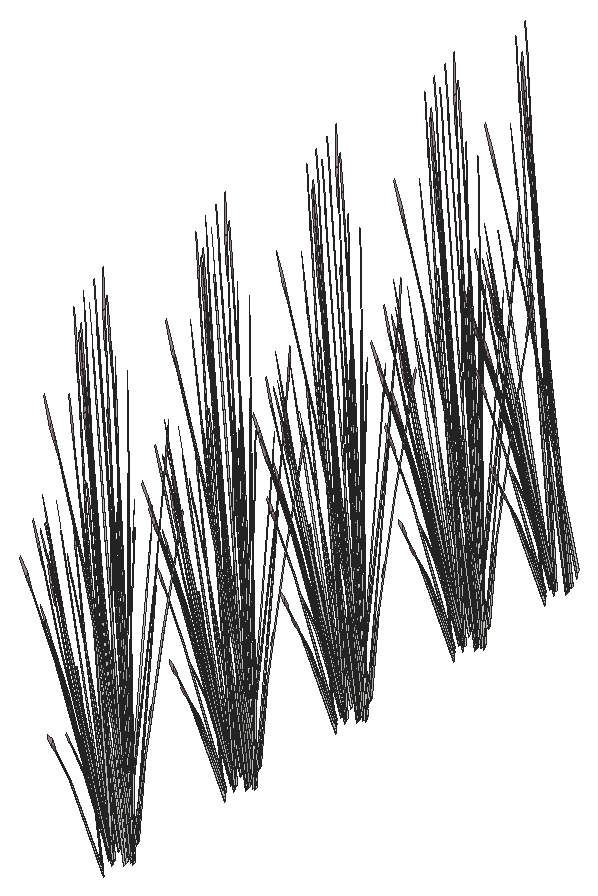
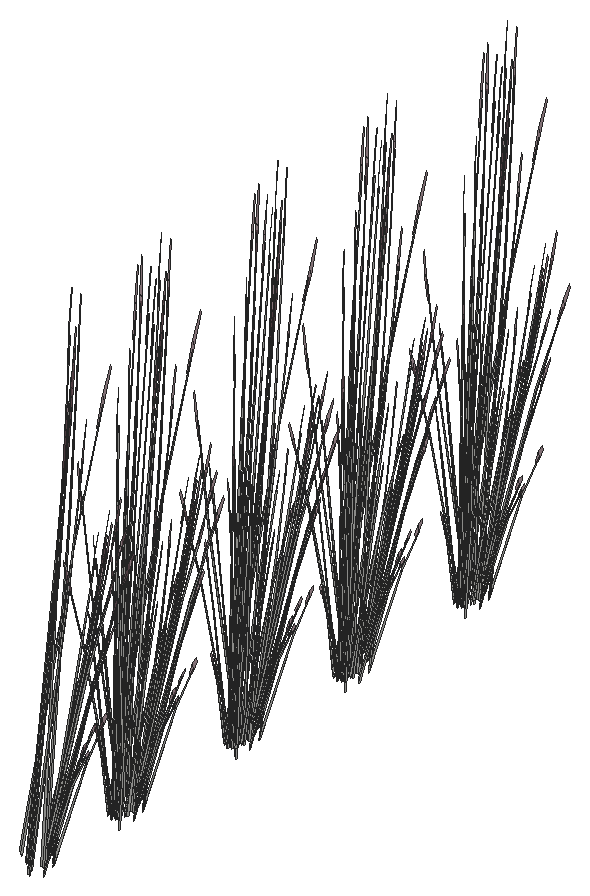
# SketchUp Ruby script. Lengths in inches.
U = 1.inch
M = Sketchup.active_model
def pt(a) = Geom::Point3d.new(a.map { |v| v * U })
def face(e, loops, mat)
  f = e.add_face(loops[0].map { |a| pt(a) })
  loops[1..].each { |l| e.add_face(l.map { |a| pt(a) }).erase! }
  f.material = f.back_material = mat if mat
  f
end
# faces: each face lists its corners as indices into pts; further lists are holes
def faces(e, pts, list, mat = nil) = list.each { |f| face(e, (f[0].is_a?(Array) ? f : [f]).map { |l| l.map { |i| pts[i] } }, mat) }
# xy, xz, yz: faces in a plane at the given z, y or x. An outline is a flat list of corners, or four numbers for a rectangle; further outlines are holes
def ring(l) = l.size == 4 ? [[l[0], l[1]], [l[2], l[1]], [l[2], l[3]], [l[0], l[3]]] : l.each_slice(2).to_a
def flat(e, list, mat, &to3) = list.each { |f| face(e, (f[0].is_a?(Array) ? f : [f]).map { |l| ring(l).map { |u, v| to3.(u, v) } }, mat) }
def xy(e, z, list, mat = nil) = flat(e, list, mat) { |x, y| [x, y, z] }
def xz(e, y, list, mat = nil) = flat(e, list, mat) { |x, z| [x, y, z] }
def yz(e, x, list, mat = nil) = flat(e, list, mat) { |y, z| [x, y, z] }
def lines(e, pts, list) = list.each { |a, b| e.add_line(pt(pts[a]), pt(pts[b])) }
# prism: a flat outline (further loops are holes) pulled along v
def prism(e, loops, v, mat = nil)
  f = face(e, loops, mat); d = Geom::Vector3d.new(v.map { |x| x * U })
  f.pushpull(f.normal.samedirection?(d) ? d.length : -d.length)
end
def box(e, o, s, mat = nil) = prism(e, [[o, [o[0] + s[0], o[1], o[2]], [o[0] + s[0], o[1] + s[1], o[2]], [o[0], o[1] + s[1], o[2]]]], [0, 0, s[2]], mat)
def at(x, y, z, deg = 0) = Geom::Transformation.translation(pt([x, y, z])) * Geom::Transformation.rotation(ORIGIN, Z_AXIS, deg.degrees)
def axes(o, x, y, z) = Geom::Transformation.new([*x, 0, *y, 0, *z, 0, *pt(o).to_a, 1])
def part(name) = M.definitions.add(name)
# library, detail: a bought-in or finely detailed component or shape, given as its bounding box
def library(name, o, s) = part(name).tap { |d| box(d.entities, o, s) }
def detail(e, o, s) = box(e.add_group.entities, o, s)
def put(e, d, t, mat = nil) = e.add_instance(d, t).tap { |i| i.material = mat if mat }
def group(e, t, mat = nil) = e.add_group.tap { |g| g.transformation = t; g.material = mat if mat }.entities
root = M.entities
M.materials.add("LightPink_Translucent").color = [144, 107, 117]
M.materials["LightPink_Translucent"].alpha = 0.75
c1 = part("blade")
p = [[2.15,0.21,22],[0,0.17,0],[0.09,0.45,0],[2.18,0.31,22],[2.29,0.31,22],[0.38,0.45,0],
  [2.48,0.24,33],[2.49,0.24,33],[2.48,0.22,33]]
faces(c1.entities,p,[[0,1,2,3],[4,5,2,3],[6,3,4,7],[8,0,3,6]])
c2 = part("seeds")
p = [[0.3,-0.1,1.38],[-0.01,-0.03,1.59],[-0.01,-0.03,0.03],[0.14,-0.07,-0.07],[0.29,-0.03,3],[0.15,0.01,3.11]]
faces(c2.entities,p,[[0,1,2,3],[1,0,4,5]],"LightPink_Translucent")
c3 = part("blade with seeds")
put(c3.entities,c1,at(0,0,0))
put(c3.entities,c2,axes([2.4,0.25,30.99],[1.5799,-0.05474,1.17369],[-0.12525,1.92788,0.29478],[-0.07173,-0.02425,1.56792]))
put(root,c3,axes([401.51,688.86,4.98],[-0.30095,-0.22541,-0.71045],[0.21388,-0.395,0.08574],[-0.10904,-0.13459,1.00501]))
put(root,c3,axes([401.4,688.56,4.53],[-0.05451,-0.37564,-0.35414],[0.31161,-0.09919,0.4572],[-0.0837,-0.10765,0.87481]))
put(root,c3,axes([400.92,688.49,1.49],[-0.03419,0.06144,1.76342],[-0.3455,0.13246,-0.26939],[-0.08346,-0.12049,0.30037]))
put(root,c3,axes([400.73,689.1,3.875],[0.1311,0.08035,1.71376],[-0.27131,0.33708,0.13857],[-0.16909,-0.15206,0.73262]))
put(root,c3,axes([401.37,688.87,4.68],[-0.34827,0.11086,-0.51099],[-0.06092,-0.41983,-0.3958],[-0.09354,-0.12031,0.97773]))
put(root,c3,axes([402.23,691.41,3.33],[0.305,0.18805,1.51261],[-0.29879,0.40513,0.59816],[-0.13384,-0.24012,1.26806]))
put(root,c3,axes([400.68,689.22,4.53],[-0.20082,-0.29199,-0.35414],[0.2293,-0.2764,0.4572],[-0.1165,-0.04206,0.87481]))
put(root,c3,axes([400.7,688.72,2.13],[-0.10181,0.3808,-0.03893],[-0.31336,-0.11714,-0.17649],[-0.04758,-0.06228,0.58215]))
put(root,c3,axes([400.53,690.46,2.375],[-0.44133,0,0],[0,-0.52122,-0.51607],[0,-0.11871,1.63711]))
put(root,c3,axes([400.61,689.53,2.59],[0.06891,0.12984,1.43002],[-0.15879,0.35293,-0.30754],[-0.16304,-0.08436,0.61141]))
put(root,c3,axes([400.89,689.41,4.98],[-0.35281,-0.01123,-0.71045],[0.0237,-0.47284,0.08574],[-0.14947,-0.0499,1.00501]))
put(root,c3,axes([400.875,690.32,2.33],[-0.32829,0.39208,0.30756],[-0.32849,-0.38796,-0.36492],[-0.01146,-0.11134,1.64885]))
put(root,c3,axes([401.77,691.14,2.4375],[0.09355,-0.55261,-0.23429],[0.44354,0.09633,0.51271],[-0.0775,-0.07631,1.5644]))
put(root,c3,axes([400.78,689.51,4.68],[-0.25628,0.30892,-0.51099],[-0.22444,-0.32634,-0.3958],[-0.13021,-0.047,0.97773]))
put(root,c3,axes([400.2,689.92,2.77],[0.22533,-0.03337,1.1486],[-0.14293,0.29403,0.84392],[-0.11135,-0.04411,0.25299]))
put(root,c3,axes([400.46,689.84,3.875],[0.14639,-0.01056,1.71376],[-0.09712,0.45778,0.13857],[-0.20862,-0.02831,0.73262]))
put(root,c3,axes([401.73,690.92,2.21],[-0.21202,-0.39143,-0.44739],[0.32115,-0.27564,0.21531],[-0.06861,-0.04843,1.43643]))
put(root,c3,axes([401.54,691.07,2.06],[-0.36714,-0.07646,-0.62353],[0.07747,-0.47163,-0.16365],[-0.10956,-0.05715,1.37633]))
put(root,c3,axes([400.36,690.4,1.49],[0.00895,0.0735,1.76342],[-0.18044,0.38382,-0.26939],[-0.12817,-0.01935,0.30037]))
put(root,c3,axes([401.15,691.78,2.03],[-0.08291,-0.40636,-0.30978],[0.32928,-0.11539,0.30978],[-0.06638,-0.04686,1.38974]))
put(root,c3,axes([401.0625,691.96,2.02],[-0.33032,-0.23318,-0.49651],[0.19744,-0.41812,0],[-0.07523,-0.05311,1.57504]))
put(root,c3,axes([400.33,690.23,4.53],[-0.29332,-0.1301,-0.35414],[0.08555,-0.37955,0.4572],[-0.11809,0.0348,0.87481]))
put(root,c3,axes([401.96,691.14,2.67],[-0.35635,0.30962,-0.29095],[-0.23697,-0.43749,-0.50002],[-0.08792,-0.04443,1.59708]))
put(root,c3,axes([401.93,691.27,2.62],[-0.06809,0.4162,0.1448],[-0.33266,-0.07225,-0.41347],[-0.06054,-0.04274,1.26744]))
put(root,c3,axes([401.22,690.17,3.34],[0.10032,-0.06746,1.77064],[0.0346,0.47103,0.13857],[-0.2173,0.0625,0.63284]))
put(root,c3,axes([402.36,691.28,2.46],[-0.34464,-0.37536,-0.25192],[0.29,-0.42149,0.5513],[-0.0928,0.04391,1.68216]))
put(root,c3,axes([401.45,692,2.48],[0.33032,0.23318,0.49651],[-0.19744,0.41812,0],[-0.07523,-0.05311,1.57504]))
put(root,c3,axes([400.53,690.43,4.68],[-0.09562,0.42421,-0.51099],[-0.32782,-0.1454,-0.3958],[-0.13199,0.0389,0.97773]))
put(root,c3,axes([401.26,692.24,2.375],[-0.22066,0.46731,0],[-0.36918,-0.26061,-0.51607],[-0.08408,-0.05936,1.63711]))
put(root,c3,axes([402.1875,691.2,2.21],[-0.38326,0.02879,-0.44739],[-0.03466,-0.47788,0.21531],[-0.06861,0.04843,1.43643]))
put(root,c3,axes([400.52,690.65,3.875],[0.12246,-0.09864,1.71376],[0.1031,0.45582,0.13857],[-0.19225,0.10302,0.73262]))
put(root,c3,axes([400.14,691.42,2.59],[0.12266,0.03828,1.43002],[0.07906,0.39104,-0.30754],[-0.16661,0.0732,0.61141]))
put(root,c3,axes([399.88,692.24,2.77],[0.14709,-0.21136,1.1486],[0.05804,0.3346,0.84392],[-0.1063,0.05991,0.25299]))
put(root,c3,axes([400.43,691.33,4.53],[-0.30722,0.06665,-0.35414],[-0.08112,-0.381,0.4572],[-0.08804,0.10234,0.87481]))
put(root,c3,axes([402.2,691.47,2.06],[-0.23773,0.35053,-0.62353],[-0.29532,-0.31785,-0.16365],[-0.09526,0.08744,1.37633]))
put(root,c3,axes([400.97,690.95,3.875],[0.08815,-0.14329,1.71376],[0.22258,0.38678,0.13857],[-0.15267,0.17614,0.73262]))
put(root,c3,axes([400.6875,691.37,4.68],[0.09067,0.42583,-0.51099],[-0.34336,0.07449,-0.3958],[-0.0984,0.11438,0.97773]))
put(root,c3,axes([400.27,692.46,1.49],[0.04734,0.04659,1.76342],[0.08027,0.4317,-0.26939],[-0.10492,0.09206,0.30037]))
put(root,c3,axes([400.9,691.31,3.875],[0.06572,-0.16029,1.71376],[0.27569,0.33172,0.13857],[-0.12437,0.20675,0.73262]))
put(root,c3,axes([400.98,692.21,4.53],[-0.23881,0.24554,-0.35414],[-0.22606,-0.28036,0.4572],[-0.0344,0.14245,0.87481]))
put(root,c3,axes([401.13,693.16,2.77],[-0.00913,-0.2773,1.1486],[0.22824,0.19778,0.84392],[-0.04489,0.13217,0.25299]))
put(root,c3,axes([401.13,691.95,5.34],[-0.00918,0.43138,-0.7886],[-0.38672,-0.02897,0.09517],[-0.04081,0.18275,1.11556]))
put(root,c3,axes([400.86,692.92,2.59],[0.11138,-0.07357,1.43002],[0.27499,0.22183,-0.30754],[-0.08185,0.19194,0.61141]))
put(root,c3,axes([401.01,692.56,3.36],[0.00775,-0.24075,1.54345],[0.34877,0.12716,0.21329],[-0.03022,0.25658,0.72882]))
put(root,c3,axes([401.27,706.37,3.875],[0.08068,0.14973,1.71376],[-0.3728,0.12606,0.13857],[-0.08426,-0.23506,0.73262]))
put(root,c3,axes([401.17,705.97,2.59],[-0.02137,0.15256,1.43002],[-0.31245,0.12771,-0.30754],[-0.07303,-0.19719,0.61141]))
put(root,c3,axes([401.0625,705.72,2.77],[0.18411,0.16231,1.1486],[-0.26813,0.09757,0.84392],[-0.05737,-0.12474,0.25299]))
put(root,c3,axes([401.51,706.58,4.98],[-0.30095,-0.22541,-0.71045],[0.21388,-0.395,0.08574],[-0.10904,-0.13459,1.00501]))
put(root,c3,axes([401.4,706.29,4.53],[-0.05451,-0.37564,-0.35414],[0.31161,-0.09919,0.4572],[-0.0837,-0.10765,0.87481]))
put(root,c3,axes([400.92,706.21,1.49],[-0.03419,0.06144,1.76342],[-0.3455,0.13246,-0.26939],[-0.08346,-0.12049,0.30037]))
put(root,c3,axes([400.73,706.83,3.875],[0.1311,0.08035,1.71376],[-0.27131,0.33708,0.13857],[-0.16909,-0.15206,0.73262]))
put(root,c3,axes([401.37,706.6,4.68],[-0.34827,0.11086,-0.51099],[-0.06092,-0.41983,-0.3958],[-0.09354,-0.12031,0.97773]))
put(root,c3,axes([402.23,709.13,3.33],[0.305,0.18805,1.51261],[-0.29879,0.40513,0.59816],[-0.13384,-0.24012,1.26806]))
put(root,c3,axes([400.68,706.95,4.53],[-0.20082,-0.29199,-0.35414],[0.2293,-0.2764,0.4572],[-0.1165,-0.04206,0.87481]))
put(root,c3,axes([400.7,706.45,2.13],[-0.10181,0.3808,-0.03893],[-0.31336,-0.11714,-0.17649],[-0.04758,-0.06228,0.58215]))
put(root,c3,axes([400.53,708.1875,2.375],[-0.44133,0,0],[0,-0.52122,-0.51607],[0,-0.11871,1.63711]))
put(root,c3,axes([400.61,707.26,2.59],[0.06891,0.12984,1.43002],[-0.15879,0.35293,-0.30754],[-0.16304,-0.08436,0.61141]))
put(root,c3,axes([400.89,707.14,4.98],[-0.35281,-0.01123,-0.71045],[0.0237,-0.47284,0.08574],[-0.14947,-0.0499,1.00501]))
put(root,c3,axes([400.875,708.05,2.33],[-0.32829,0.39208,0.30756],[-0.32849,-0.38796,-0.36492],[-0.01146,-0.11134,1.64885]))
put(root,c3,axes([401.77,708.87,2.4375],[0.09355,-0.55261,-0.23429],[0.44354,0.09633,0.51271],[-0.0775,-0.07631,1.5644]))
put(root,c3,axes([400.78,707.24,4.68],[-0.25628,0.30892,-0.51099],[-0.22444,-0.32634,-0.3958],[-0.13021,-0.047,0.97773]))
put(root,c3,axes([400.2,707.65,2.77],[0.22533,-0.03337,1.1486],[-0.14293,0.29403,0.84392],[-0.11135,-0.04411,0.25299]))
put(root,c3,axes([400.46,707.57,3.875],[0.14639,-0.01056,1.71376],[-0.09712,0.45778,0.13857],[-0.20862,-0.02831,0.73262]))
put(root,c3,axes([401.73,708.64,2.21],[-0.21202,-0.39143,-0.44739],[0.32115,-0.27564,0.21531],[-0.06861,-0.04843,1.43643]))
put(root,c3,axes([401.54,708.79,2.06],[-0.36714,-0.07646,-0.62353],[0.07747,-0.47163,-0.16365],[-0.10956,-0.05715,1.37633]))
put(root,c3,axes([400.36,708.13,1.49],[0.00895,0.0735,1.76342],[-0.18044,0.38382,-0.26939],[-0.12817,-0.01935,0.30037]))
put(root,c3,axes([401.15,709.51,2.03],[-0.08291,-0.40636,-0.30978],[0.32928,-0.11539,0.30978],[-0.06638,-0.04686,1.38974]))
put(root,c3,axes([401.0625,709.6875,2.02],[-0.33032,-0.23318,-0.49651],[0.19744,-0.41812,0],[-0.07523,-0.05311,1.57504]))
put(root,c3,axes([400.33,707.96,4.53],[-0.29332,-0.1301,-0.35414],[0.08555,-0.37955,0.4572],[-0.11809,0.0348,0.87481]))
put(root,c3,axes([401.96,708.86,2.67],[-0.35635,0.30962,-0.29095],[-0.23697,-0.43749,-0.50002],[-0.08792,-0.04443,1.59708]))
put(root,c3,axes([401.93,709,2.62],[-0.06809,0.4162,0.1448],[-0.33266,-0.07225,-0.41347],[-0.06054,-0.04274,1.26744]))
put(root,c3,axes([401.22,707.9,3.34],[0.10032,-0.06746,1.77064],[0.0346,0.47103,0.13857],[-0.2173,0.0625,0.63284]))
put(root,c3,axes([402.36,709,2.46],[-0.34464,-0.37536,-0.25192],[0.29,-0.42149,0.5513],[-0.0928,0.04391,1.68216]))
put(root,c3,axes([401.45,709.72,2.48],[0.33032,0.23318,0.49651],[-0.19744,0.41812,0],[-0.07523,-0.05311,1.57504]))
put(root,c3,axes([400.53,708.15,4.68],[-0.09562,0.42421,-0.51099],[-0.32782,-0.1454,-0.3958],[-0.13199,0.0389,0.97773]))
put(root,c3,axes([401.26,709.97,2.375],[-0.22066,0.46731,0],[-0.36918,-0.26061,-0.51607],[-0.08408,-0.05936,1.63711]))
put(root,c3,axes([402.1875,708.92,2.21],[-0.38326,0.02879,-0.44739],[-0.03466,-0.47788,0.21531],[-0.06861,0.04843,1.43643]))
put(root,c3,axes([400.52,708.37,3.875],[0.12246,-0.09864,1.71376],[0.1031,0.45582,0.13857],[-0.19225,0.10302,0.73262]))
put(root,c3,axes([400.14,709.15,2.59],[0.12266,0.03828,1.43002],[0.07906,0.39104,-0.30754],[-0.16661,0.0732,0.61141]))
put(root,c3,axes([399.88,709.97,2.77],[0.14709,-0.21136,1.1486],[0.05804,0.3346,0.84392],[-0.1063,0.05991,0.25299]))
put(root,c3,axes([400.43,709.05,4.53],[-0.30722,0.06665,-0.35414],[-0.08112,-0.381,0.4572],[-0.08804,0.10234,0.87481]))
put(root,c3,axes([402.2,709.2,2.06],[-0.23773,0.35053,-0.62353],[-0.29532,-0.31785,-0.16365],[-0.09526,0.08744,1.37633]))
put(root,c3,axes([400.97,708.68,3.875],[0.08815,-0.14329,1.71376],[0.22258,0.38678,0.13857],[-0.15267,0.17614,0.73262]))
put(root,c3,axes([400.6875,709.1,4.68],[0.09067,0.42583,-0.51099],[-0.34336,0.07449,-0.3958],[-0.0984,0.11438,0.97773]))
put(root,c3,axes([400.27,710.1875,1.49],[0.04734,0.04659,1.76342],[0.08027,0.4317,-0.26939],[-0.10492,0.09206,0.30037]))
put(root,c3,axes([400.9,709.03,3.875],[0.06572,-0.16029,1.71376],[0.27569,0.33172,0.13857],[-0.12437,0.20675,0.73262]))
put(root,c3,axes([400.98,709.9375,4.53],[-0.23881,0.24554,-0.35414],[-0.22606,-0.28036,0.4572],[-0.0344,0.14245,0.87481]))
put(root,c3,axes([401.13,710.89,2.77],[-0.00913,-0.2773,1.1486],[0.22824,0.19778,0.84392],[-0.04489,0.13217,0.25299]))
put(root,c3,axes([401.13,709.68,5.34],[-0.00918,0.43138,-0.7886],[-0.38672,-0.02897,0.09517],[-0.04081,0.18275,1.11556]))
put(root,c3,axes([400.86,710.64,2.59],[0.11138,-0.07357,1.43002],[0.27499,0.22183,-0.30754],[-0.08185,0.19194,0.61141]))
put(root,c3,axes([401.01,710.28,3.36],[0.00775,-0.24075,1.54345],[0.34877,0.12716,0.21329],[-0.03022,0.25658,0.72882]))
put(root,c3,axes([401.27,722.48,3.875],[0.08068,0.14973,1.71376],[-0.3728,0.12606,0.13857],[-0.08426,-0.23506,0.73262]))
put(root,c3,axes([401.17,722.08,2.59],[-0.02137,0.15256,1.43002],[-0.31245,0.12771,-0.30754],[-0.07303,-0.19719,0.61141]))
put(root,c3,axes([401.0625,721.83,2.77],[0.18411,0.16231,1.1486],[-0.26813,0.09757,0.84392],[-0.05737,-0.12474,0.25299]))
put(root,c3,axes([401.51,722.7,4.98],[-0.30095,-0.22541,-0.71045],[0.21388,-0.395,0.08574],[-0.10904,-0.13459,1.00501]))
put(root,c3,axes([401.4,722.4,4.53],[-0.05451,-0.37564,-0.35414],[0.31161,-0.09919,0.4572],[-0.0837,-0.10765,0.87481]))
put(root,c3,axes([400.92,722.32,1.49],[-0.03419,0.06144,1.76342],[-0.3455,0.13246,-0.26939],[-0.08346,-0.12049,0.30037]))
put(root,c3,axes([400.73,722.94,3.875],[0.1311,0.08035,1.71376],[-0.27131,0.33708,0.13857],[-0.16909,-0.15206,0.73262]))
put(root,c3,axes([401.37,722.71,4.68],[-0.34827,0.11086,-0.51099],[-0.06092,-0.41983,-0.3958],[-0.09354,-0.12031,0.97773]))
put(root,c3,axes([402.23,725.25,3.33],[0.305,0.18805,1.51261],[-0.29879,0.40513,0.59816],[-0.13384,-0.24012,1.26806]))
put(root,c3,axes([400.68,723.06,4.53],[-0.20082,-0.29199,-0.35414],[0.2293,-0.2764,0.4572],[-0.1165,-0.04206,0.87481]))
put(root,c3,axes([400.7,722.5625,2.13],[-0.10181,0.3808,-0.03893],[-0.31336,-0.11714,-0.17649],[-0.04758,-0.06228,0.58215]))
put(root,c3,axes([400.53,724.3,2.375],[-0.44133,0,0],[0,-0.52122,-0.51607],[0,-0.11871,1.63711]))
put(root,c3,axes([400.61,723.37,2.59],[0.06891,0.12984,1.43002],[-0.15879,0.35293,-0.30754],[-0.16304,-0.08436,0.61141]))
put(root,c3,axes([400.89,723.25,4.98],[-0.35281,-0.01123,-0.71045],[0.0237,-0.47284,0.08574],[-0.14947,-0.0499,1.00501]))
put(root,c3,axes([400.875,724.16,2.33],[-0.32829,0.39208,0.30756],[-0.32849,-0.38796,-0.36492],[-0.01146,-0.11134,1.64885]))
put(root,c3,axes([401.77,724.98,2.4375],[0.09355,-0.55261,-0.23429],[0.44354,0.09633,0.51271],[-0.0775,-0.07631,1.5644]))
put(root,c3,axes([400.78,723.35,4.68],[-0.25628,0.30892,-0.51099],[-0.22444,-0.32634,-0.3958],[-0.13021,-0.047,0.97773]))
put(root,c3,axes([400.2,723.76,2.77],[0.22533,-0.03337,1.1486],[-0.14293,0.29403,0.84392],[-0.11135,-0.04411,0.25299]))
put(root,c3,axes([400.46,723.68,3.875],[0.14639,-0.01056,1.71376],[-0.09712,0.45778,0.13857],[-0.20862,-0.02831,0.73262]))
put(root,c3,axes([401.73,724.75,2.21],[-0.21202,-0.39143,-0.44739],[0.32115,-0.27564,0.21531],[-0.06861,-0.04843,1.43643]))
put(root,c3,axes([401.54,724.9,2.06],[-0.36714,-0.07646,-0.62353],[0.07747,-0.47163,-0.16365],[-0.10956,-0.05715,1.37633]))
put(root,c3,axes([400.36,724.24,1.49],[0.00895,0.0735,1.76342],[-0.18044,0.38382,-0.26939],[-0.12817,-0.01935,0.30037]))
put(root,c3,axes([401.15,725.625,2.03],[-0.08291,-0.40636,-0.30978],[0.32928,-0.11539,0.30978],[-0.06638,-0.04686,1.38974]))
put(root,c3,axes([401.0625,725.8,2.02],[-0.33032,-0.23318,-0.49651],[0.19744,-0.41812,0],[-0.07523,-0.05311,1.57504]))
put(root,c3,axes([400.33,724.07,4.53],[-0.29332,-0.1301,-0.35414],[0.08555,-0.37955,0.4572],[-0.11809,0.0348,0.87481]))
put(root,c3,axes([401.96,724.97,2.67],[-0.35635,0.30962,-0.29095],[-0.23697,-0.43749,-0.50002],[-0.08792,-0.04443,1.59708]))
put(root,c3,axes([401.93,725.11,2.62],[-0.06809,0.4162,0.1448],[-0.33266,-0.07225,-0.41347],[-0.06054,-0.04274,1.26744]))
put(root,c3,axes([401.22,724.01,3.34],[0.10032,-0.06746,1.77064],[0.0346,0.47103,0.13857],[-0.2173,0.0625,0.63284]))
put(root,c3,axes([402.36,725.12,2.46],[-0.34464,-0.37536,-0.25192],[0.29,-0.42149,0.5513],[-0.0928,0.04391,1.68216]))
put(root,c3,axes([401.45,725.83,2.48],[0.33032,0.23318,0.49651],[-0.19744,0.41812,0],[-0.07523,-0.05311,1.57504]))
put(root,c3,axes([400.53,724.26,4.68],[-0.09562,0.42421,-0.51099],[-0.32782,-0.1454,-0.3958],[-0.13199,0.0389,0.97773]))
put(root,c3,axes([401.26,726.08,2.375],[-0.22066,0.46731,0],[-0.36918,-0.26061,-0.51607],[-0.08408,-0.05936,1.63711]))
put(root,c3,axes([402.1875,725.04,2.21],[-0.38326,0.02879,-0.44739],[-0.03466,-0.47788,0.21531],[-0.06861,0.04843,1.43643]))
put(root,c3,axes([400.52,724.48,3.875],[0.12246,-0.09864,1.71376],[0.1031,0.45582,0.13857],[-0.19225,0.10302,0.73262]))
put(root,c3,axes([400.14,725.26,2.59],[0.12266,0.03828,1.43002],[0.07906,0.39104,-0.30754],[-0.16661,0.0732,0.61141]))
put(root,c3,axes([399.88,726.08,2.77],[0.14709,-0.21136,1.1486],[0.05804,0.3346,0.84392],[-0.1063,0.05991,0.25299]))
put(root,c3,axes([400.43,725.17,4.53],[-0.30722,0.06665,-0.35414],[-0.08112,-0.381,0.4572],[-0.08804,0.10234,0.87481]))
put(root,c3,axes([402.2,725.3125,2.06],[-0.23773,0.35053,-0.62353],[-0.29532,-0.31785,-0.16365],[-0.09526,0.08744,1.37633]))
put(root,c3,axes([400.97,724.79,3.875],[0.08815,-0.14329,1.71376],[0.22258,0.38678,0.13857],[-0.15267,0.17614,0.73262]))
put(root,c3,axes([400.6875,725.21,4.68],[0.09067,0.42583,-0.51099],[-0.34336,0.07449,-0.3958],[-0.0984,0.11438,0.97773]))
put(root,c3,axes([400.27,726.3,1.49],[0.04734,0.04659,1.76342],[0.08027,0.4317,-0.26939],[-0.10492,0.09206,0.30037]))
put(root,c3,axes([400.9,725.14,3.875],[0.06572,-0.16029,1.71376],[0.27569,0.33172,0.13857],[-0.12437,0.20675,0.73262]))
put(root,c3,axes([400.98,726.05,4.53],[-0.23881,0.24554,-0.35414],[-0.22606,-0.28036,0.4572],[-0.0344,0.14245,0.87481]))
put(root,c3,axes([401.13,727,2.77],[-0.00913,-0.2773,1.1486],[0.22824,0.19778,0.84392],[-0.04489,0.13217,0.25299]))
put(root,c3,axes([401.13,725.79,5.34],[-0.00918,0.43138,-0.7886],[-0.38672,-0.02897,0.09517],[-0.04081,0.18275,1.11556]))
put(root,c3,axes([400.86,726.76,2.59],[0.11138,-0.07357,1.43002],[0.27499,0.22183,-0.30754],[-0.08185,0.19194,0.61141]))
put(root,c3,axes([401.01,726.4,3.36],[0.00775,-0.24075,1.54345],[0.34877,0.12716,0.21329],[-0.03022,0.25658,0.72882]))
put(root,c3,axes([401.27,739.62,3.875],[0.08068,0.14973,1.71376],[-0.3728,0.12606,0.13857],[-0.08426,-0.23506,0.73262]))
put(root,c3,axes([401.17,739.23,2.59],[-0.02137,0.15256,1.43002],[-0.31245,0.12771,-0.30754],[-0.07303,-0.19719,0.61141]))
put(root,c3,axes([401.0625,738.98,2.77],[0.18411,0.16231,1.1486],[-0.26813,0.09757,0.84392],[-0.05737,-0.12474,0.25299]))
put(root,c3,axes([401.51,739.84,4.98],[-0.30095,-0.22541,-0.71045],[0.21388,-0.395,0.08574],[-0.10904,-0.13459,1.00501]))
put(root,c3,axes([401.4,739.54,4.53],[-0.05451,-0.37564,-0.35414],[0.31161,-0.09919,0.4572],[-0.0837,-0.10765,0.87481]))
put(root,c3,axes([400.92,739.47,1.49],[-0.03419,0.06144,1.76342],[-0.3455,0.13246,-0.26939],[-0.08346,-0.12049,0.30037]))
put(root,c3,axes([400.73,740.09,3.875],[0.1311,0.08035,1.71376],[-0.27131,0.33708,0.13857],[-0.16909,-0.15206,0.73262]))
put(root,c3,axes([401.37,739.85,4.68],[-0.34827,0.11086,-0.51099],[-0.06092,-0.41983,-0.3958],[-0.09354,-0.12031,0.97773]))
put(root,c3,axes([402.23,742.39,3.33],[0.305,0.18805,1.51261],[-0.29879,0.40513,0.59816],[-0.13384,-0.24012,1.26806]))
put(root,c3,axes([400.68,740.2,4.53],[-0.20082,-0.29199,-0.35414],[0.2293,-0.2764,0.4572],[-0.1165,-0.04206,0.87481]))
put(root,c3,axes([400.7,739.71,2.13],[-0.10181,0.3808,-0.03893],[-0.31336,-0.11714,-0.17649],[-0.04758,-0.06228,0.58215]))
put(root,c3,axes([400.53,741.45,2.375],[-0.44133,0,0],[0,-0.52122,-0.51607],[0,-0.11871,1.63711]))
put(root,c3,axes([400.61,740.51,2.59],[0.06891,0.12984,1.43002],[-0.15879,0.35293,-0.30754],[-0.16304,-0.08436,0.61141]))
put(root,c3,axes([400.89,740.4,4.98],[-0.35281,-0.01123,-0.71045],[0.0237,-0.47284,0.08574],[-0.14947,-0.0499,1.00501]))
put(root,c3,axes([400.875,741.31,2.33],[-0.32829,0.39208,0.30756],[-0.32849,-0.38796,-0.36492],[-0.01146,-0.11134,1.64885]))
put(root,c3,axes([401.77,742.125,2.4375],[0.09355,-0.55261,-0.23429],[0.44354,0.09633,0.51271],[-0.0775,-0.07631,1.5644]))
put(root,c3,axes([400.78,740.5,4.68],[-0.25628,0.30892,-0.51099],[-0.22444,-0.32634,-0.3958],[-0.13021,-0.047,0.97773]))
put(root,c3,axes([400.2,740.9,2.77],[0.22533,-0.03337,1.1486],[-0.14293,0.29403,0.84392],[-0.11135,-0.04411,0.25299]))
put(root,c3,axes([400.46,740.82,3.875],[0.14639,-0.01056,1.71376],[-0.09712,0.45778,0.13857],[-0.20862,-0.02831,0.73262]))
put(root,c3,axes([401.73,741.9,2.21],[-0.21202,-0.39143,-0.44739],[0.32115,-0.27564,0.21531],[-0.06861,-0.04843,1.43643]))
put(root,c3,axes([401.54,742.05,2.06],[-0.36714,-0.07646,-0.62353],[0.07747,-0.47163,-0.16365],[-0.10956,-0.05715,1.37633]))
put(root,c3,axes([400.36,741.38,1.49],[0.00895,0.0735,1.76342],[-0.18044,0.38382,-0.26939],[-0.12817,-0.01935,0.30037]))
put(root,c3,axes([401.15,742.77,2.03],[-0.08291,-0.40636,-0.30978],[0.32928,-0.11539,0.30978],[-0.06638,-0.04686,1.38974]))
put(root,c3,axes([401.0625,742.94,2.02],[-0.33032,-0.23318,-0.49651],[0.19744,-0.41812,0],[-0.07523,-0.05311,1.57504]))
put(root,c3,axes([400.33,741.22,4.53],[-0.29332,-0.1301,-0.35414],[0.08555,-0.37955,0.4572],[-0.11809,0.0348,0.87481]))
put(root,c3,axes([401.96,742.12,2.67],[-0.35635,0.30962,-0.29095],[-0.23697,-0.43749,-0.50002],[-0.08792,-0.04443,1.59708]))
put(root,c3,axes([401.93,742.26,2.62],[-0.06809,0.4162,0.1448],[-0.33266,-0.07225,-0.41347],[-0.06054,-0.04274,1.26744]))
put(root,c3,axes([401.22,741.15,3.34],[0.10032,-0.06746,1.77064],[0.0346,0.47103,0.13857],[-0.2173,0.0625,0.63284]))
put(root,c3,axes([402.36,742.26,2.46],[-0.34464,-0.37536,-0.25192],[0.29,-0.42149,0.5513],[-0.0928,0.04391,1.68216]))
put(root,c3,axes([401.45,742.98,2.48],[0.33032,0.23318,0.49651],[-0.19744,0.41812,0],[-0.07523,-0.05311,1.57504]))
put(root,c3,axes([400.53,741.41,4.68],[-0.09562,0.42421,-0.51099],[-0.32782,-0.1454,-0.3958],[-0.13199,0.0389,0.97773]))
put(root,c3,axes([401.26,743.23,2.375],[-0.22066,0.46731,0],[-0.36918,-0.26061,-0.51607],[-0.08408,-0.05936,1.63711]))
put(root,c3,axes([402.1875,742.18,2.21],[-0.38326,0.02879,-0.44739],[-0.03466,-0.47788,0.21531],[-0.06861,0.04843,1.43643]))
put(root,c3,axes([400.52,741.63,3.875],[0.12246,-0.09864,1.71376],[0.1031,0.45582,0.13857],[-0.19225,0.10302,0.73262]))
put(root,c3,axes([400.14,742.41,2.59],[0.12266,0.03828,1.43002],[0.07906,0.39104,-0.30754],[-0.16661,0.0732,0.61141]))
put(root,c3,axes([399.88,743.23,2.77],[0.14709,-0.21136,1.1486],[0.05804,0.3346,0.84392],[-0.1063,0.05991,0.25299]))
put(root,c3,axes([400.43,742.3125,4.53],[-0.30722,0.06665,-0.35414],[-0.08112,-0.381,0.4572],[-0.08804,0.10234,0.87481]))
put(root,c3,axes([402.2,742.46,2.06],[-0.23773,0.35053,-0.62353],[-0.29532,-0.31785,-0.16365],[-0.09526,0.08744,1.37633]))
put(root,c3,axes([400.97,741.9375,3.875],[0.08815,-0.14329,1.71376],[0.22258,0.38678,0.13857],[-0.15267,0.17614,0.73262]))
put(root,c3,axes([400.6875,742.36,4.68],[0.09067,0.42583,-0.51099],[-0.34336,0.07449,-0.3958],[-0.0984,0.11438,0.97773]))
put(root,c3,axes([400.27,743.44,1.49],[0.04734,0.04659,1.76342],[0.08027,0.4317,-0.26939],[-0.10492,0.09206,0.30037]))
put(root,c3,axes([400.9,742.29,3.875],[0.06572,-0.16029,1.71376],[0.27569,0.33172,0.13857],[-0.12437,0.20675,0.73262]))
put(root,c3,axes([400.98,743.19,4.53],[-0.23881,0.24554,-0.35414],[-0.22606,-0.28036,0.4572],[-0.0344,0.14245,0.87481]))
put(root,c3,axes([401.13,744.15,2.77],[-0.00913,-0.2773,1.1486],[0.22824,0.19778,0.84392],[-0.04489,0.13217,0.25299]))
put(root,c3,axes([401.13,742.93,5.34],[-0.00918,0.43138,-0.7886],[-0.38672,-0.02897,0.09517],[-0.04081,0.18275,1.11556]))
put(root,c3,axes([400.86,743.9,2.59],[0.11138,-0.07357,1.43002],[0.27499,0.22183,-0.30754],[-0.08185,0.19194,0.61141]))
put(root,c3,axes([401.01,743.54,3.36],[0.00775,-0.24075,1.54345],[0.34877,0.12716,0.21329],[-0.03022,0.25658,0.72882]))
put(root,c3,axes([401.27,752.85,3.875],[0.08068,0.14973,1.71376],[-0.3728,0.12606,0.13857],[-0.08426,-0.23506,0.73262]))
put(root,c3,axes([401.17,752.46,2.59],[-0.02137,0.15256,1.43002],[-0.31245,0.12771,-0.30754],[-0.07303,-0.19719,0.61141]))
put(root,c3,axes([401.0625,752.21,2.77],[0.18411,0.16231,1.1486],[-0.26813,0.09757,0.84392],[-0.05737,-0.12474,0.25299]))
put(root,c3,axes([401.51,753.07,4.98],[-0.30095,-0.22541,-0.71045],[0.21388,-0.395,0.08574],[-0.10904,-0.13459,1.00501]))
put(root,c3,axes([401.4,752.77,4.53],[-0.05451,-0.37564,-0.35414],[0.31161,-0.09919,0.4572],[-0.0837,-0.10765,0.87481]))
put(root,c3,axes([400.92,752.7,1.49],[-0.03419,0.06144,1.76342],[-0.3455,0.13246,-0.26939],[-0.08346,-0.12049,0.30037]))
put(root,c3,axes([400.73,753.32,3.875],[0.1311,0.08035,1.71376],[-0.27131,0.33708,0.13857],[-0.16909,-0.15206,0.73262]))
put(root,c3,axes([401.37,753.08,4.68],[-0.34827,0.11086,-0.51099],[-0.06092,-0.41983,-0.3958],[-0.09354,-0.12031,0.97773]))
put(root,c3,axes([402.23,755.62,3.33],[0.305,0.18805,1.51261],[-0.29879,0.40513,0.59816],[-0.13384,-0.24012,1.26806]))
put(root,c3,axes([400.68,753.43,4.53],[-0.20082,-0.29199,-0.35414],[0.2293,-0.2764,0.4572],[-0.1165,-0.04206,0.87481]))
put(root,c3,axes([400.7,752.9375,2.13],[-0.10181,0.3808,-0.03893],[-0.31336,-0.11714,-0.17649],[-0.04758,-0.06228,0.58215]))
put(root,c3,axes([400.53,754.68,2.375],[-0.44133,0,0],[0,-0.52122,-0.51607],[0,-0.11871,1.63711]))
put(root,c3,axes([400.61,753.74,2.59],[0.06891,0.12984,1.43002],[-0.15879,0.35293,-0.30754],[-0.16304,-0.08436,0.61141]))
put(root,c3,axes([400.89,753.63,4.98],[-0.35281,-0.01123,-0.71045],[0.0237,-0.47284,0.08574],[-0.14947,-0.0499,1.00501]))
put(root,c3,axes([400.875,754.54,2.33],[-0.32829,0.39208,0.30756],[-0.32849,-0.38796,-0.36492],[-0.01146,-0.11134,1.64885]))
put(root,c3,axes([401.77,755.36,2.4375],[0.09355,-0.55261,-0.23429],[0.44354,0.09633,0.51271],[-0.0775,-0.07631,1.5644]))
put(root,c3,axes([400.78,753.72,4.68],[-0.25628,0.30892,-0.51099],[-0.22444,-0.32634,-0.3958],[-0.13021,-0.047,0.97773]))
put(root,c3,axes([400.2,754.13,2.77],[0.22533,-0.03337,1.1486],[-0.14293,0.29403,0.84392],[-0.11135,-0.04411,0.25299]))
put(root,c3,axes([400.46,754.05,3.875],[0.14639,-0.01056,1.71376],[-0.09712,0.45778,0.13857],[-0.20862,-0.02831,0.73262]))
put(root,c3,axes([401.73,755.13,2.21],[-0.21202,-0.39143,-0.44739],[0.32115,-0.27564,0.21531],[-0.06861,-0.04843,1.43643]))
put(root,c3,axes([401.54,755.28,2.06],[-0.36714,-0.07646,-0.62353],[0.07747,-0.47163,-0.16365],[-0.10956,-0.05715,1.37633]))
put(root,c3,axes([400.36,754.61,1.49],[0.00895,0.0735,1.76342],[-0.18044,0.38382,-0.26939],[-0.12817,-0.01935,0.30037]))
put(root,c3,axes([401.15,756,2.03],[-0.08291,-0.40636,-0.30978],[0.32928,-0.11539,0.30978],[-0.06638,-0.04686,1.38974]))
put(root,c3,axes([401.0625,756.17,2.02],[-0.33032,-0.23318,-0.49651],[0.19744,-0.41812,0],[-0.07523,-0.05311,1.57504]))
